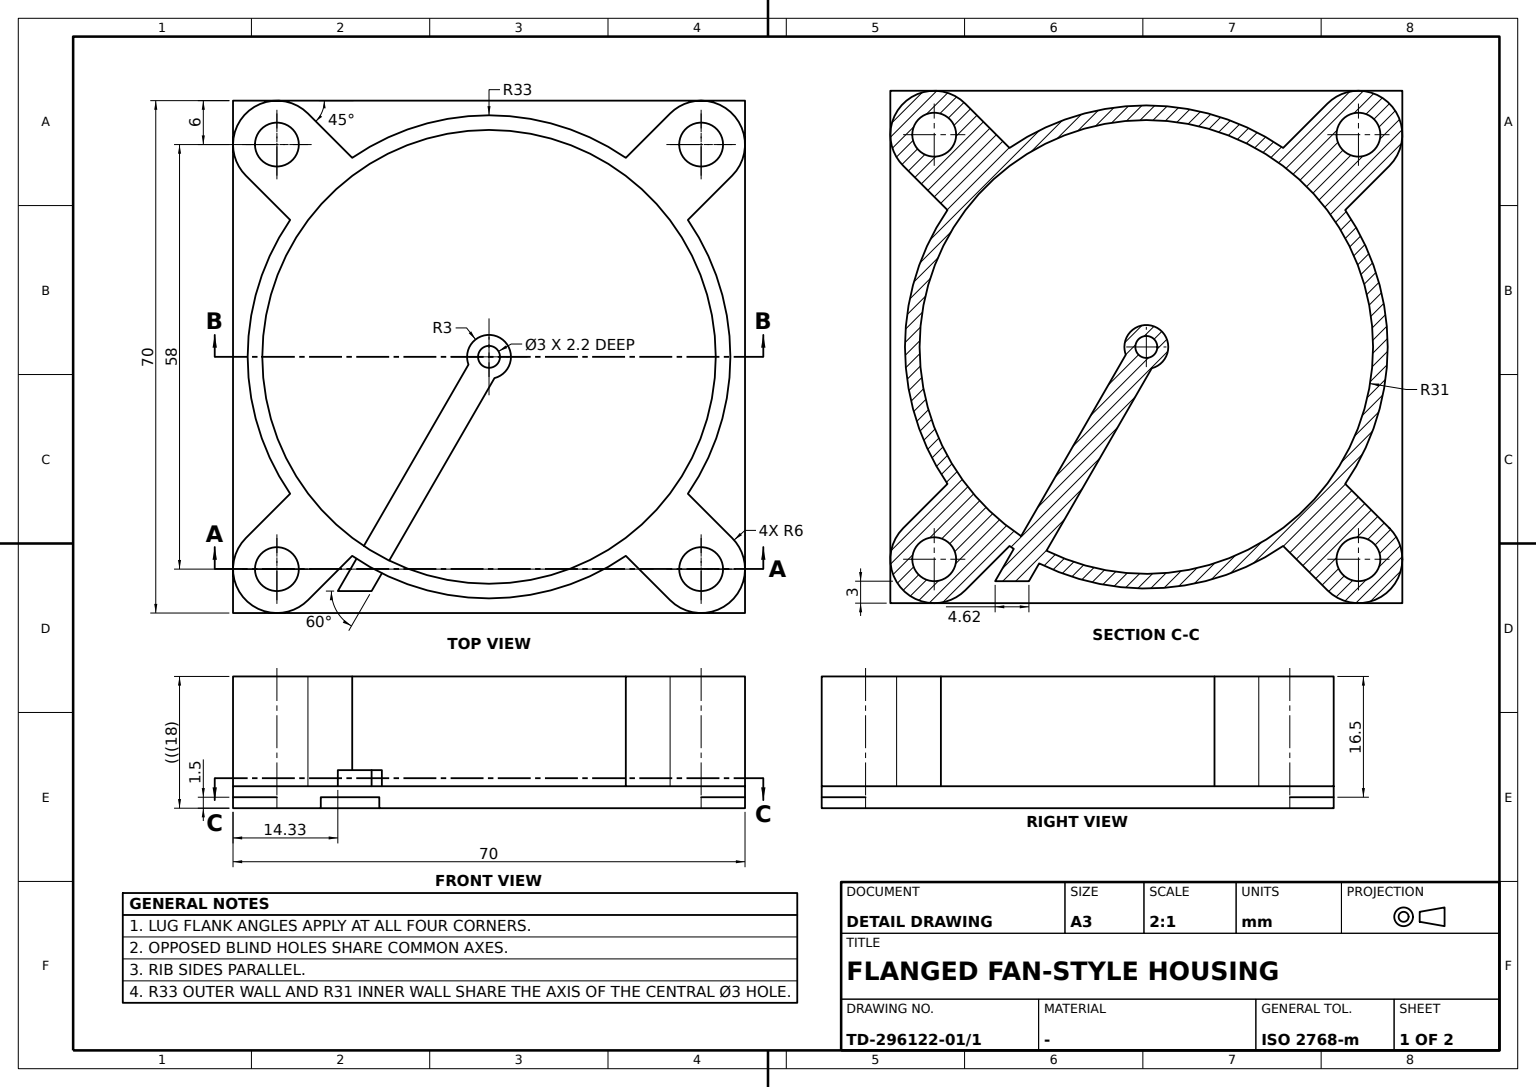
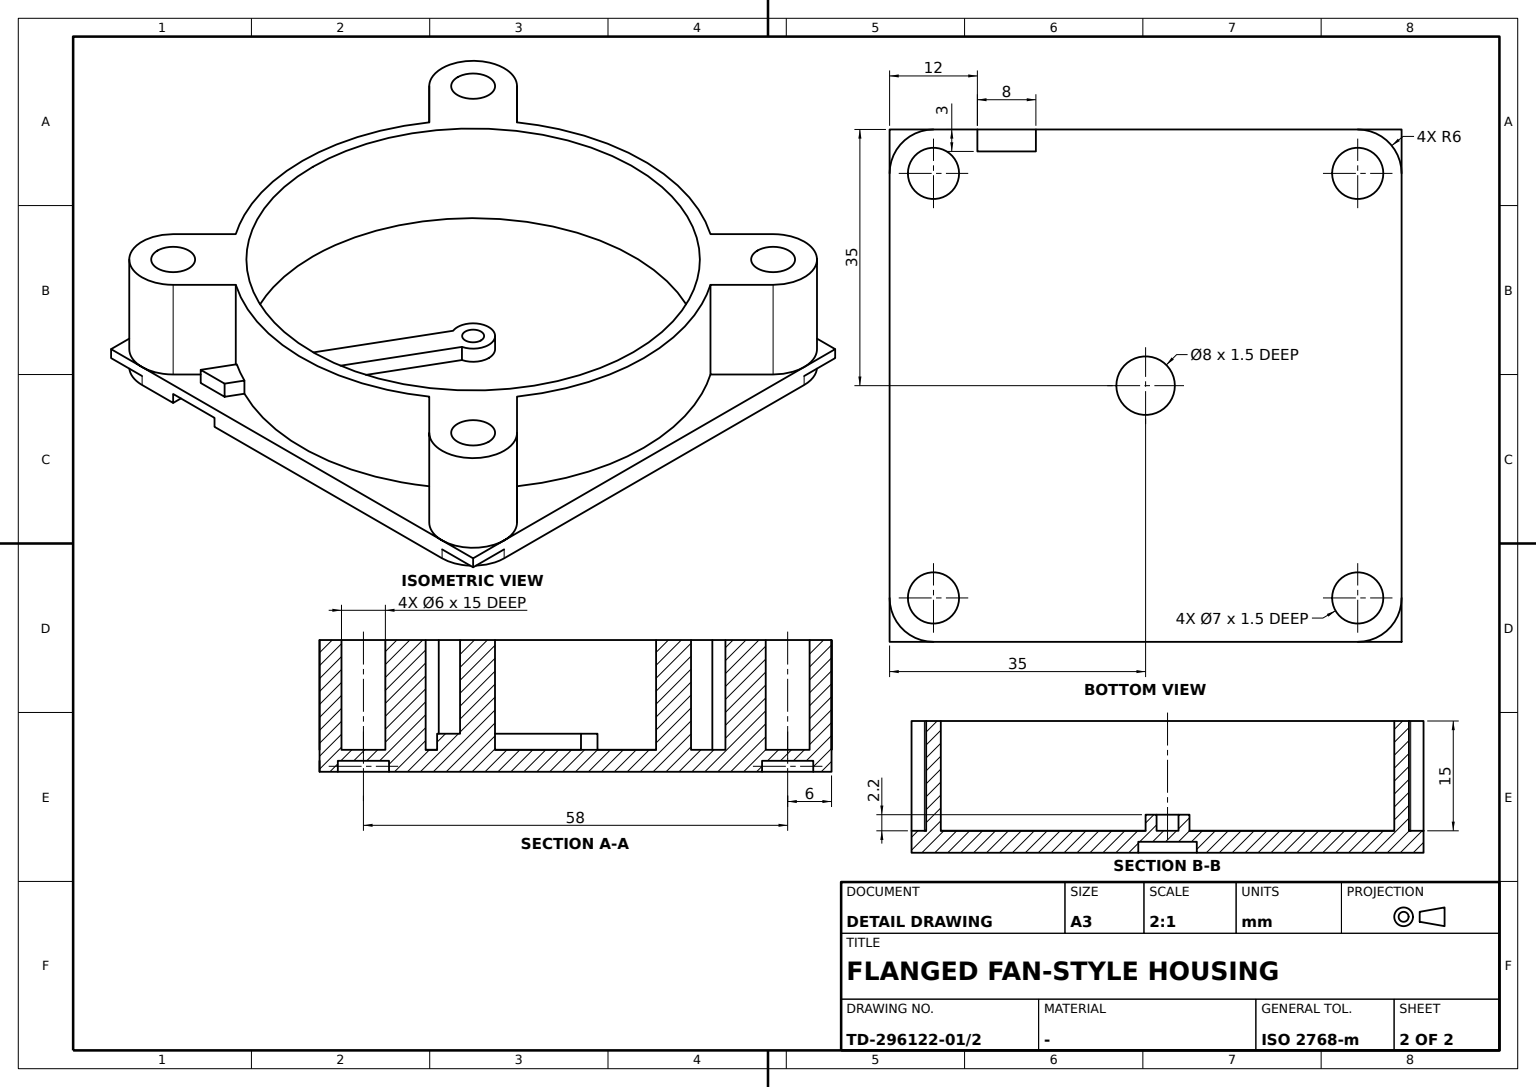
solid
v1 (26,29,3)
v2 (26,29,18)
e1 v1 v2 LINE
v3 (32,29,3)
e2 v3 v1 CIRCLE(AX(P(29,29,3),D(0,0,1),D(1,0,0)),3)
v4 (32,29,18)
e3 v3 v4 LINE
e4 v4 v2 CIRCLE(AX(P(29,29,18),D(0,0,1),D(1,0,0)),3)
face CYL(AX(P(29,29,9.75),D(0,0,-1),D(1,0,0)),3) rev [-e1 -e2 e3 e4]
v5 (29,35,3)
v6 (-29,35,3)
e5 v5 v6 LINE
v7 (-24.757359,33.242641,3)
e6 v7 v6 CIRCLE(AX(P(-29,29,3),D(0,0,1),D(1,0,0)),6)
v8 (-18.702947,27.188228,3)
e7 v7 v8 LINE
v9 (18.702947,27.188228,3)
e8 v9 v8 CIRCLE(AX(P(0,0,3),D(0,0,1),D(1,0,0)),33)
v10 (24.757359,33.242641,3)
e9 v9 v10 LINE
e10 v5 v10 CIRCLE(AX(P(29,29,3),D(0,0,1),D(1,0,0)),6)
face PLANE(AX(P(0,0,3),D(0,0,1),D(1,0,0))) [e5 -e6 e7 -e8 e9 -e10]
v11 (25.5,-29,1.5)
v12 (32.5,-29,1.5)
e11 v11 v12 CIRCLE(AX(P(29,-29,1.5),D(0,0,1),D(1,0,0)),3.5)
e12 v12 v11 CIRCLE(AX(P(29,-29,1.5),D(0,0,1),D(1,0,0)),3.5)
face PLANE(AX(P(0,0,1.5),D(0,0,1),D(1,0,0))) rev [-e11 -e12]
v13 (-25.5,29,1.5)
v14 (-32.5,29,1.5)
e13 v13 v14 CIRCLE(AX(P(-29,29,1.5),D(0,0,1),D(1,0,0)),3.5)
v15 (-32.5,29,0)
e14 v14 v15 LINE
v16 (-25.5,29,0)
e15 v16 v15 CIRCLE(AX(P(-29,29,0),D(0,0,1),D(1,0,0)),3.5)
e16 v13 v16 LINE
face CYL(AX(P(-29,29,0.5),D(0,0,-1),D(1,0,0)),3.5) rev [e13 e14 -e15 -e16]
v17 (35,-29,18)
v18 (33.242641,-24.757359,18)
e17 v17 v18 CIRCLE(AX(P(29,-29,18),D(0,0,1),D(1,0,0)),6)
v19 (35,-29,3)
e18 v17 v19 LINE
v20 (33.242641,-24.757359,3)
e19 v19 v20 CIRCLE(AX(P(29,-29,3),D(0,0,1),D(1,0,0)),6)
e20 v20 v18 LINE
face CYL(AX(P(29,-29,0.75),D(0,0,-1),D(1,0,0)),6) [-e17 e18 e19 e20]
e21 v1 v3 CIRCLE(AX(P(29,29,3),D(0,0,1),D(1,0,0)),3)
face PLANE(AX(P(0,0,3),D(0,0,1),D(1,0,0))) [e21 e2]
v21 (29,-35,1.5)
v22 (35,-29,1.5)
e22 v21 v22 CIRCLE(AX(P(29,-29,1.5),D(0,0,1),D(1,0,0)),6)
v23 (35,-35,1.5)
e23 v23 v22 LINE
e24 v21 v23 LINE
face PLANE(AX(P(0,0,1.5),D(0,0,1),D(1,0,0))) rev [e22 -e23 -e24]
v24 (-35,29,3)
v25 (-33.242641,24.757359,3)
e25 v24 v25 CIRCLE(AX(P(-29,29,3),D(0,0,1),D(1,0,0)),6)
v26 (-33.242641,24.757359,18)
e26 v25 v26 LINE
v27 (-35,29,18)
e27 v27 v26 CIRCLE(AX(P(-29,29,18),D(0,0,1),D(-1,0,0)),6)
e28 v27 v24 LINE
face CYL(AX(P(-29,29,0.75),D(0,0,-1),D(-1,0,0)),6) [e25 e26 -e27 e28]
v28 (33.242641,24.757359,18)
v29 (29,35,18)
e29 v28 v29 CIRCLE(AX(P(29,29,18),D(0,0,1),D(0,1,0)),6)
v30 (33.242641,24.757359,3)
e30 v30 v28 LINE
v31 (35,29,3)
e31 v30 v31 CIRCLE(AX(P(29,29,3),D(0,0,1),D(1,0,0)),6)
e32 v31 v5 CIRCLE(AX(P(29,29,3),D(0,0,1),D(1,0,0)),6)
e33 v29 v5 LINE
face CYL(AX(P(29,29,0.75),D(0,0,-1),D(0,1,0)),6) [-e29 -e30 e31 e32 -e33]
v32 (-24.757359,33.242641,18)
e34 v32 v27 CIRCLE(AX(P(-29,29,18),D(0,0,1),D(-1,0,0)),6)
e35 v7 v32 LINE
e36 v6 v24 CIRCLE(AX(P(-29,29,3),D(0,0,1),D(1,0,0)),6)
face CYL(AX(P(-29,29,0.75),D(0,0,-1),D(-1,0,0)),6) [-e34 -e35 e6 e36 -e28]
v33 (-29,-35,0)
v34 (-23,-35,0)
e37 v33 v34 LINE
v35 (-35,-29,0)
e38 v35 v33 CIRCLE(AX(P(-29,-29,0),D(0,0,1),D(1,0,0)),6)
v36 (-35,29,0)
e39 v36 v35 LINE
v37 (-29,35,0)
e40 v37 v36 CIRCLE(AX(P(-29,29,0),D(0,0,1),D(1,0,0)),6)
v38 (29,35,0)
e41 v38 v37 LINE
v39 (35,29,0)
e42 v39 v38 CIRCLE(AX(P(29,29,0),D(0,0,1),D(1,0,0)),6)
v40 (35,-29,0)
e43 v40 v39 LINE
v41 (29,-35,0)
e44 v41 v40 CIRCLE(AX(P(29,-29,0),D(0,0,1),D(1,0,0)),6)
v42 (-15,-35,0)
e45 v42 v41 LINE
v43 (-15,-32,0)
e46 v42 v43 LINE
v44 (-23,-32,0)
e47 v44 v43 LINE
e48 v34 v44 LINE
v45 (-25.5,-29,0)
v46 (-32.5,-29,0)
e49 v45 v46 CIRCLE(AX(P(-29,-29,0),D(0,0,1),D(1,0,0)),3.5)
e50 v46 v45 CIRCLE(AX(P(-29,-29,0),D(0,0,1),D(1,0,0)),3.5)
v47 (-4,0,0)
v48 (4,0,0)
e51 v47 v48 CIRCLE(AX(P(0,0,0),D(0,0,-1),D(1,0,0)),4)
e52 v48 v47 CIRCLE(AX(P(0,0,0),D(0,0,-1),D(1,0,0)),4)
v49 (25.5,29,0)
v50 (32.5,29,0)
e53 v49 v50 CIRCLE(AX(P(29,29,0),D(0,0,1),D(1,0,0)),3.5)
e54 v50 v49 CIRCLE(AX(P(29,29,0),D(0,0,1),D(1,0,0)),3.5)
e55 v15 v16 CIRCLE(AX(P(-29,29,0),D(0,0,1),D(1,0,0)),3.5)
v51 (25.5,-29,0)
v52 (32.5,-29,0)
e56 v51 v52 CIRCLE(AX(P(29,-29,0),D(0,0,1),D(1,0,0)),3.5)
e57 v52 v51 CIRCLE(AX(P(29,-29,0),D(0,0,1),D(1,0,0)),3.5)
face PLANE(AX(P(0,0,0),D(0,0,1),D(1,0,0))) rev [-e37 -e38 -e39 -e40 -e41 -e42 -e43 -e44 -e45 e46 -e47 -e48] [e49 e50] [-e51 -e52] [e53 e54] [e55 e15] [e56 e57]
v53 (-18.702947,27.188228,18)
e58 v53 v32 LINE
e59 v8 v53 LINE
face PLANE(AX(P(27.188228,-18.702947,1.5),D(-0.707106781,-0.707106781,0),D(0.707106781,-0.707106781,0))) rev [-e7 e35 -e58 -e59]
v54 (-15,-35,1.5)
e60 v54 v42 LINE
e61 v41 v21 LINE
v55 (35,-35,3)
e62 v23 v55 LINE
v56 (29,-35,3)
e63 v56 v55 LINE
v57 (-29,-35,3)
e64 v57 v56 LINE
v58 (-35,-35,3)
e65 v58 v57 LINE
v59 (-35,-35,1.5)
e66 v59 v58 LINE
v60 (-29,-35,1.5)
e67 v59 v60 LINE
e68 v33 v60 LINE
v61 (-23,-35,1.5)
e69 v61 v34 LINE
e70 v61 v54 LINE
face PLANE(AX(P(35,-35,0),D(0,1,0),D(-1,0,0))) rev [e60 e45 e61 e24 e62 -e63 -e64 -e65 -e66 e67 -e68 e37 -e69 e70]
v62 (4,0,1.5)
e71 v48 v62 LINE
v63 (-4,0,1.5)
e72 v47 v63 LINE
e73 v62 v63 CIRCLE(AX(P(0,0,1.5),D(0,0,-1),D(1,0,0)),4)
face CYL(AX(P(0,0,0.75),D(0,0,1),D(1,0,0)),4) rev [-e71 e52 e72 -e73]
v64 (18.702947,27.188228,18)
e74 v9 v64 LINE
v65 (24.757359,33.242641,18)
e75 v65 v64 LINE
e76 v10 v65 LINE
face PLANE(AX(P(18.702947,27.188228,1.5),D(0.707106781,-0.707106781,0),D(0.707106781,0.707106781,0))) rev [-e9 e74 -e75 -e76]
v66 (31,0,3)
v67 (31,0,18)
e77 v66 v67 LINE
v68 (-13.64759,-27.834211,3)
e78 v68 v66 CIRCLE(AX(P(0,0,3),D(0,0,1),D(1,0,0)),31)
v69 (-13.64759,-27.834211,5.2)
e79 v69 v68 LINE
v70 (-17.118024,-25.845178,5.2)
e80 v70 v69 CIRCLE(AX(P(0,0,5.2),D(0,0,1),D(1,0,0)),31)
v71 (-17.118024,-25.845178,3)
e81 v70 v71 LINE
v72 (-31,0,3)
e82 v72 v71 CIRCLE(AX(P(0,0,3),D(0,0,1),D(1,0,0)),31)
v73 (-31,0,18)
e83 v72 v73 LINE
e84 v73 v67 CIRCLE(AX(P(0,0,18),D(0,0,1),D(1,0,0)),31)
face CYL(AX(P(0,0,9.75),D(0,0,-1),D(1,0,0)),31) rev [-e77 -e78 -e79 -e80 e81 -e82 e83 e84]
e85 v63 v62 CIRCLE(AX(P(0,0,1.5),D(0,0,-1),D(1,0,0)),4)
face CYL(AX(P(0,0,0.75),D(0,0,1),D(1,0,0)),4) rev [-e85 -e72 e51 e71]
v74 (-35,35,3)
e86 v6 v74 LINE
e87 v74 v24 LINE
face PLANE(AX(P(0,0,3),D(0,0,1),D(1,0,0))) [e86 e87 -e36]
v75 (29,35,1.5)
e88 v38 v75 LINE
v76 (35,29,1.5)
e89 v76 v75 CIRCLE(AX(P(29,29,1.5),D(0,0,1),D(1,0,0)),6)
e90 v39 v76 LINE
face CYL(AX(P(29,29,0.75),D(0,0,-1),D(0,1,0)),6) [e88 -e89 -e90 e42]
v77 (35,35,1.5)
e91 v76 v77 LINE
e92 v77 v75 LINE
face PLANE(AX(P(0,0,1.5),D(0,0,1),D(1,0,0))) rev [-e91 e89 -e92]
v78 (3,0,3)
v79 (-3,0,3)
e93 v78 v79 CIRCLE(AX(P(0,0,3),D(0,0,1),D(1,0,0)),3)
v80 (-3,0,5.2)
e94 v79 v80 LINE
v81 (3,0,5.2)
e95 v81 v80 CIRCLE(AX(P(0,0,5.2),D(0,0,1),D(1,0,0)),3)
e96 v78 v81 LINE
face CYL(AX(P(0,0,4.1),D(0,0,-1),D(1,0,0)),3) [e93 e94 -e95 -e96]
v82 (-35,-29,3)
e97 v24 v82 LINE
v83 (-35,35,1.5)
e98 v83 v74 LINE
v84 (-35,29,1.5)
e99 v83 v84 LINE
e100 v36 v84 LINE
v85 (-35,-29,1.5)
e101 v35 v85 LINE
e102 v85 v59 LINE
e103 v82 v58 LINE
face PLANE(AX(P(-35,-35,0),D(1,0,0),D(0,1,0))) rev [-e97 -e87 -e98 e99 -e100 e39 e101 e102 e66 -e103]
v86 (-33.242641,-24.757359,3)
e104 v86 v82 CIRCLE(AX(P(-29,-29,3),D(0,0,1),D(1,0,0)),6)
e105 v82 v57 CIRCLE(AX(P(-29,-29,3),D(0,0,1),D(1,0,0)),6)
v87 (-29,-35,18)
e106 v87 v57 LINE
v88 (-33.242641,-24.757359,18)
e107 v88 v87 CIRCLE(AX(P(-29,-29,18),D(0,0,1),D(0,-1,0)),6)
e108 v86 v88 LINE
face CYL(AX(P(-29,-29,0.75),D(0,0,-1),D(0,-1,0)),6) [e104 e105 -e106 -e107 -e108]
v89 (-14.649748,-29.569999,3)
v90 (18.702947,-27.188228,3)
e109 v89 v90 CIRCLE(AX(P(0,0,3),D(0,0,1),D(1,0,0)),33)
v91 (18.702947,-27.188228,18)
e110 v90 v91 LINE
v92 (-18.702947,-27.188228,18)
e111 v92 v91 CIRCLE(AX(P(0,0,18),D(0,0,1),D(1,0,0)),33)
v93 (-18.702947,-27.188228,3)
e112 v93 v92 LINE
v94 (-18.119797,-27.5803,3)
e113 v93 v94 CIRCLE(AX(P(0,0,3),D(0,0,1),D(1,0,0)),33)
v95 (-18.119797,-27.5803,5.2)
e114 v95 v94 LINE
v96 (-14.649748,-29.569999,5.2)
e115 v95 v96 CIRCLE(AX(P(0,0,5.2),D(0,0,1),D(1,0,0)),33)
e116 v96 v89 LINE
face CYL(AX(P(0,0,9.75),D(0,0,-1),D(1,0,0)),33) [e109 e110 -e111 -e112 e113 -e114 e115 e116]
v97 (-24.757359,-33.242641,3)
e117 v57 v97 CIRCLE(AX(P(-29,-29,3),D(0,0,1),D(1,0,0)),6)
v98 (-24.757359,-33.242641,18)
e118 v97 v98 LINE
e119 v87 v98 CIRCLE(AX(P(-29,-29,18),D(0,0,1),D(0,-1,0)),6)
face CYL(AX(P(-29,-29,0.75),D(0,0,-1),D(0,-1,0)),6) [e106 e117 e118 -e119]
v99 (33,0,3)
v100 (33,0,18)
e120 v99 v100 LINE
v101 (27.188228,-18.702947,18)
e121 v101 v100 CIRCLE(AX(P(0,0,18),D(0,0,1),D(1,0,0)),33)
v102 (27.188228,-18.702947,3)
e122 v102 v101 LINE
e123 v102 v99 CIRCLE(AX(P(0,0,3),D(0,0,1),D(1,0,0)),33)
face CYL(AX(P(0,0,9.75),D(0,0,-1),D(1,0,0)),33) [e120 -e121 -e122 e123]
e124 v55 v19 LINE
e125 v56 v19 CIRCLE(AX(P(29,-29,3),D(0,0,1),D(1,0,0)),6)
face PLANE(AX(P(0,0,3),D(0,0,1),D(1,0,0))) [e63 e124 -e125]
v103 (-1.5,0,3)
v104 (1.5,0,3)
e126 v103 v104 CIRCLE(AX(P(0,0,3),D(0,0,1),D(1,0,0)),1.5)
v105 (-1.5,0,5.2)
e127 v105 v103 LINE
v106 (1.5,0,5.2)
e128 v105 v106 CIRCLE(AX(P(0,0,5.2),D(0,0,1),D(1,0,0)),1.5)
e129 v106 v104 LINE
face CYL(AX(P(0,0,-7.55),D(0,0,-1),D(1,0,0)),1.5) rev [-e126 -e127 e128 e129]
v107 (-27.188228,18.702947,3)
v108 (-27.188228,18.702947,18)
e130 v107 v108 LINE
v109 (-33,0,3)
e131 v107 v109 CIRCLE(AX(P(0,0,3),D(0,0,1),D(1,0,0)),33)
v110 (-33,0,18)
e132 v109 v110 LINE
e133 v108 v110 CIRCLE(AX(P(0,0,18),D(0,0,1),D(1,0,0)),33)
face CYL(AX(P(0,0,9.75),D(0,0,-1),D(1,0,0)),33) [-e130 e131 e132 -e133]
v111 (-23,-32,1.5)
e134 v111 v44 LINE
e135 v61 v111 LINE
face PLANE(AX(P(-23,-32,5.2),D(1,0,0),D(0,-1,0))) [-e134 -e135 e69 e48]
v112 (-25.5,-29,1.5)
e136 v112 v45 LINE
v113 (-32.5,-29,1.5)
e137 v112 v113 CIRCLE(AX(P(-29,-29,1.5),D(0,0,1),D(1,0,0)),3.5)
e138 v113 v46 LINE
face CYL(AX(P(-29,-29,0.5),D(0,0,-1),D(1,0,0)),3.5) rev [-e49 -e136 e137 e138]
v114 (-15,-32,1.5)
e139 v114 v43 LINE
e140 v111 v114 LINE
face PLANE(AX(P(-23,-32,5.2),D(0,1,0),D(1,0,0))) rev [-e139 -e140 e134 e47]
v115 (24.757359,-33.242641,18)
e141 v115 v17 CIRCLE(AX(P(29,-29,18),D(0,0,1),D(1,0,0)),6)
v116 (24.757359,-33.242641,3)
e142 v116 v115 LINE
e143 v116 v56 CIRCLE(AX(P(29,-29,3),D(0,0,1),D(1,0,0)),6)
face CYL(AX(P(29,-29,0.75),D(0,0,-1),D(1,0,0)),6) [e125 -e18 -e141 -e142 e143]
v117 (35,35,3)
e144 v31 v117 LINE
e145 v19 v31 LINE
e146 v40 v22 LINE
e147 v77 v117 LINE
face PLANE(AX(P(35,35,0),D(-1,0,0),D(0,-1,0))) rev [-e144 -e145 -e124 -e62 e23 -e146 e43 e90 e91 e147]
v118 (-29,35,1.5)
e148 v37 v118 LINE
e149 v118 v83 LINE
e150 v117 v5 LINE
face PLANE(AX(P(-35,35,0),D(0,-1,0),D(1,0,0))) rev [e92 -e88 e41 e148 e149 e98 -e86 -e5 -e150 -e147]
v119 (-26,29,3)
v120 (-32,29,3)
e151 v119 v120 CIRCLE(AX(P(-29,29,3),D(0,0,1),D(1,0,0)),3)
e152 v120 v119 CIRCLE(AX(P(-29,29,3),D(0,0,1),D(1,0,0)),3)
face PLANE(AX(P(0,0,3),D(0,0,1),D(1,0,0))) [e151 e152]
v121 (32.5,29,1.5)
e153 v121 v50 LINE
v122 (25.5,29,1.5)
e154 v121 v122 CIRCLE(AX(P(29,29,1.5),D(0,0,1),D(1,0,0)),3.5)
e155 v122 v49 LINE
face CYL(AX(P(29,29,0.5),D(0,0,-1),D(1,0,0)),3.5) rev [-e54 -e153 e154 e155]
e156 v113 v112 CIRCLE(AX(P(-29,-29,1.5),D(0,0,1),D(1,0,0)),3.5)
face CYL(AX(P(-29,-29,0.5),D(0,0,-1),D(1,0,0)),3.5) rev [-e50 -e138 e156 e136]
v123 (-27.188228,-18.702947,18)
e157 v110 v123 CIRCLE(AX(P(0,0,18),D(0,0,1),D(1,0,0)),33)
v124 (-27.188228,-18.702947,3)
e158 v109 v124 CIRCLE(AX(P(0,0,3),D(0,0,1),D(1,0,0)),33)
e159 v124 v123 LINE
face CYL(AX(P(0,0,9.75),D(0,0,-1),D(1,0,0)),33) [-e157 -e132 e158 e159]
v125 (-2.807205,-1.058112,3)
e160 v125 v71 LINE
v126 (-2.807205,-1.058112,5.2)
e161 v126 v70 LINE
e162 v126 v125 LINE
face PLANE(AX(P(-2.807205,-1.058112,5.2),D(0.866025404,-0.5,0),D(-0.5,-0.866025404,0))) rev [e160 -e81 -e161 e162]
v127 (-32,-29,3)
v128 (-32,-29,18)
e163 v127 v128 LINE
v129 (-26,-29,18)
e164 v128 v129 CIRCLE(AX(P(-29,-29,18),D(0,0,1),D(1,0,0)),3)
v130 (-26,-29,3)
e165 v130 v129 LINE
e166 v127 v130 CIRCLE(AX(P(-29,-29,3),D(0,0,1),D(1,0,0)),3)
face CYL(AX(P(-29,-29,9.75),D(0,0,-1),D(1,0,0)),3) rev [e163 e164 -e165 -e166]
v131 (-20.671512,-32,3)
e167 v94 v131 LINE
v132 (-20.671512,-32,5.2)
e168 v132 v131 LINE
e169 v95 v132 LINE
face PLANE(AX(P(-2.807205,-1.058112,5.2),D(0.866025404,-0.5,0),D(-0.5,-0.866025404,0))) rev [e167 -e168 -e169 e114]
v133 (0.744654,-2.906113,3)
e170 v133 v78 CIRCLE(AX(P(0,0,3),D(0,0,1),D(1,0,0)),3)
e171 v133 v68 LINE
e172 v66 v72 CIRCLE(AX(P(0,0,3),D(0,0,1),D(1,0,0)),31)
e173 v79 v125 CIRCLE(AX(P(0,0,3),D(0,0,1),D(1,0,0)),3)
face PLANE(AX(P(0,0,3),D(0,0,1),D(1,0,0))) [-e170 e171 e78 e172 e82 -e160 -e173 -e93]
e174 v67 v73 CIRCLE(AX(P(0,0,18),D(0,0,1),D(1,0,0)),31)
face CYL(AX(P(0,0,9.75),D(0,0,-1),D(1,0,0)),31) rev [-e172 e77 e174 -e83]
e175 v98 v92 LINE
e176 v97 v93 LINE
face PLANE(AX(P(27.188228,18.702947,1.5),D(0.707106781,-0.707106781,0),D(0.707106781,0.707106781,0))) [-e175 -e118 e176 e112]
e177 v85 v60 CIRCLE(AX(P(-29,-29,1.5),D(0,0,1),D(1,0,0)),6)
face PLANE(AX(P(0,0,1.5),D(0,0,1),D(1,0,0))) rev [e177 -e67 -e102]
v134 (0.744654,-2.906113,5.2)
e178 v134 v133 LINE
e179 v69 v134 LINE
face PLANE(AX(P(0.744654,-2.906113,5.2),D(0.866025404,-0.5,0),D(-0.5,-0.866025404,0))) [e79 -e171 -e178 -e179]
e180 v134 v81 CIRCLE(AX(P(0,0,5.2),D(0,0,1),D(1,0,0)),3)
face CYL(AX(P(0,0,4.1),D(0,0,-1),D(1,0,0)),3) [e96 -e180 e178 e170]
e181 v29 v65 CIRCLE(AX(P(29,29,18),D(0,0,1),D(0,1,0)),6)
e182 v64 v53 CIRCLE(AX(P(0,0,18),D(0,0,1),D(1,0,0)),33)
e183 v26 v108 LINE
e184 v123 v88 LINE
e185 v91 v115 LINE
e186 v18 v101 LINE
v135 (27.188228,18.702947,18)
e187 v100 v135 CIRCLE(AX(P(0,0,18),D(0,0,1),D(1,0,0)),33)
e188 v135 v28 LINE
v136 (-26,29,18)
v137 (-32,29,18)
e189 v136 v137 CIRCLE(AX(P(-29,29,18),D(0,0,1),D(1,0,0)),3)
e190 v137 v136 CIRCLE(AX(P(-29,29,18),D(0,0,1),D(1,0,0)),3)
e191 v2 v4 CIRCLE(AX(P(29,29,18),D(0,0,1),D(1,0,0)),3)
v138 (32,-29,18)
v139 (26,-29,18)
e192 v138 v139 CIRCLE(AX(P(29,-29,18),D(0,0,1),D(1,0,0)),3)
e193 v139 v138 CIRCLE(AX(P(29,-29,18),D(0,0,1),D(1,0,0)),3)
e194 v129 v128 CIRCLE(AX(P(-29,-29,18),D(0,0,1),D(1,0,0)),3)
face PLANE(AX(P(0,0,18),D(0,0,1),D(1,0,0))) [e29 e181 e75 e182 e58 e34 e27 e183 e133 e157 e184 e107 e119 e175 e111 e185 e141 e17 e186 e121 e187 e188] [-e189 -e190] [-e4 -e191] [-e192 -e193] [-e84 -e174] [-e194 -e164]
face CYL(AX(P(29,-29,0.75),D(0,0,-1),D(1,0,0)),6) [-e22 -e61 e44 e146]
face CYL(AX(P(0,0,9.75),D(0,0,-1),D(1,0,0)),33) [-e182 -e74 e8 e59]
v140 (-16.05271,-32,5.2)
v141 (-16.05271,-32,3)
e195 v140 v141 LINE
e196 v89 v141 LINE
e197 v140 v96 LINE
face PLANE(AX(P(0.744654,-2.906113,5.2),D(0.866025404,-0.5,0),D(-0.5,-0.866025404,0))) [e195 -e196 -e116 -e197]
e198 v86 v124 LINE
face PLANE(AX(P(18.702947,27.188228,1.5),D(0.707106781,-0.707106781,0),D(0.707106781,0.707106781,0))) rev [-e198 e108 -e184 -e159]
e199 v25 v107 LINE
face PLANE(AX(P(0,0,3),D(0,0,1),D(1,0,0))) [e97 -e104 e198 -e158 -e131 -e199 -e25]
e200 v12 v52 LINE
e201 v11 v51 LINE
face CYL(AX(P(29,-29,0.5),D(0,0,-1),D(1,0,0)),3.5) rev [-e200 e12 e201 -e57]
e202 v14 v13 CIRCLE(AX(P(-29,29,1.5),D(0,0,1),D(1,0,0)),3.5)
face PLANE(AX(P(0,0,1.5),D(0,0,1),D(1,0,0))) rev [-e202 -e13]
face PLANE(AX(P(18.702947,-27.188228,1.5),D(-0.707106781,-0.707106781,0),D(0.707106781,-0.707106781,0))) [e199 e130 -e183 -e26]
e203 v130 v127 CIRCLE(AX(P(-29,-29,3),D(0,0,1),D(1,0,0)),3)
face PLANE(AX(P(0,0,3),D(0,0,1),D(1,0,0))) [e203 e166]
v142 (26,-29,3)
v143 (32,-29,3)
e204 v142 v143 CIRCLE(AX(P(29,-29,3),D(0,0,1),D(1,0,0)),3)
e205 v143 v142 CIRCLE(AX(P(29,-29,3),D(0,0,1),D(1,0,0)),3)
face PLANE(AX(P(0,0,3),D(0,0,1),D(1,0,0))) [e204 e205]
face PLANE(AX(P(0,0,3),D(0,0,1),D(1,0,0))) [e103 e65 -e105]
e206 v54 v114 LINE
face PLANE(AX(P(0,0,1.5),D(0,0,1),D(1,0,0))) rev [-e206 -e70 e135 e140]
e207 v106 v105 CIRCLE(AX(P(0,0,5.2),D(0,0,1),D(1,0,0)),1.5)
e208 v104 v103 CIRCLE(AX(P(0,0,3),D(0,0,1),D(1,0,0)),1.5)
face CYL(AX(P(0,0,-7.55),D(0,0,-1),D(1,0,0)),1.5) rev [-e129 e207 e127 -e208]
face PLANE(AX(P(0,0,3),D(0,0,1),D(1,0,0))) [e126 e208]
e209 v131 v141 LINE
e210 v140 v132 LINE
face PLANE(AX(P(-23,-32,5.2),D(0,1,0),D(1,0,0))) rev [e209 -e195 e210 e168]
e211 v120 v137 LINE
e212 v119 v136 LINE
face CYL(AX(P(-29,29,9.75),D(0,0,-1),D(1,0,0)),3) rev [-e211 -e151 e212 e189]
face CYL(AX(P(29,29,9.75),D(0,0,-1),D(1,0,0)),3) rev [-e21 e1 e191 -e3]
e213 v143 v138 LINE
e214 v142 v139 LINE
face CYL(AX(P(29,-29,9.75),D(0,0,-1),D(1,0,0)),3) rev [e213 e192 -e214 -e205]
face PLANE(AX(P(0,0,1.5),D(0,0,1),D(1,0,0))) rev [e73 e85]
face CYL(AX(P(-29,29,0.5),D(0,0,-1),D(1,0,0)),3.5) rev [-e14 e202 e16 -e55]
e215 v90 v116 LINE
face PLANE(AX(P(18.702947,-27.188228,1.5),D(-0.707106781,-0.707106781,0),D(0.707106781,-0.707106781,0))) [-e185 -e110 e215 e142]
e216 v102 v20 LINE
face PLANE(AX(P(27.188228,-18.702947,1.5),D(-0.707106781,-0.707106781,0),D(0.707106781,-0.707106781,0))) rev [e122 -e186 -e20 -e216]
v144 (27.188228,18.702947,3)
e217 v144 v30 LINE
e218 v99 v144 CIRCLE(AX(P(0,0,3),D(0,0,1),D(1,0,0)),33)
face PLANE(AX(P(0,0,3),D(0,0,1),D(1,0,0))) [-e31 -e217 -e218 -e123 e216 -e19 e145]
e219 v122 v121 CIRCLE(AX(P(29,29,1.5),D(0,0,1),D(1,0,0)),3.5)
face CYL(AX(P(29,29,0.5),D(0,0,-1),D(1,0,0)),3.5) rev [-e155 e219 e153 -e53]
e220 v80 v126 CIRCLE(AX(P(0,0,5.2),D(0,0,1),D(1,0,0)),3)
face CYL(AX(P(0,0,4.1),D(0,0,-1),D(1,0,0)),3) [-e220 -e94 e173 -e162]
face PLANE(AX(P(0,0,3),D(0,0,1),D(1,0,0))) [e64 -e143 -e215 -e109 e196 -e209 -e167 -e113 -e176 -e117]
face PLANE(AX(P(0,0,3),D(0,0,1),D(1,0,0))) [e150 -e32 e144]
face PLANE(AX(P(0,0,1.5),D(0,0,1),D(1,0,0))) rev [-e156 -e137]
face CYL(AX(P(29,29,0.75),D(0,0,-1),D(0,1,0)),6) [e76 -e181 e33 e10]
face PLANE(AX(P(0,0,5.2),D(0,0,1),D(1,0,0))) [e220 e161 e80 e179 e180 e95] [-e128 -e207]
face CYL(AX(P(-29,-29,9.75),D(0,0,-1),D(1,0,0)),3) rev [e194 -e163 -e203 e165]
face CYL(AX(P(-29,29,9.75),D(0,0,-1),D(1,0,0)),3) rev [-e212 -e152 e211 e190]
e221 v144 v135 LINE
face CYL(AX(P(0,0,9.75),D(0,0,-1),D(1,0,0)),33) [e218 e221 -e187 -e120]
face CYL(AX(P(29,-29,9.75),D(0,0,-1),D(1,0,0)),3) rev [-e213 -e204 e214 e193]
face PLANE(AX(P(0,0,5.2),D(0,0,1),D(1,0,0))) [-e210 e197 -e115 e169]
face PLANE(AX(P(0,0,1.5),D(0,0,1),D(1,0,0))) rev [-e219 -e154]
e222 v118 v84 CIRCLE(AX(P(-29,29,1.5),D(0,0,1),D(1,0,0)),6)
face PLANE(AX(P(0,0,1.5),D(0,0,1),D(1,0,0))) rev [-e149 e222 -e99]
face CYL(AX(P(-29,-29,0.75),D(0,0,-1),D(0,-1,0)),6) [e68 -e177 -e101 e38]
face PLANE(AX(P(-15,-35,5.2),D(-1,0,0),D(0,1,0))) [e139 -e46 -e60 e206]
face CYL(AX(P(29,-29,0.5),D(0,0,-1),D(1,0,0)),3.5) rev [-e56 -e201 e11 e200]
face CYL(AX(P(-29,29,0.75),D(0,0,-1),D(-1,0,0)),6) [-e148 e40 e100 -e222]
face PLANE(AX(P(27.188228,18.702947,1.5),D(0.707106781,-0.707106781,0),D(0.707106781,0.707106781,0))) [-e221 e217 e30 -e188]
